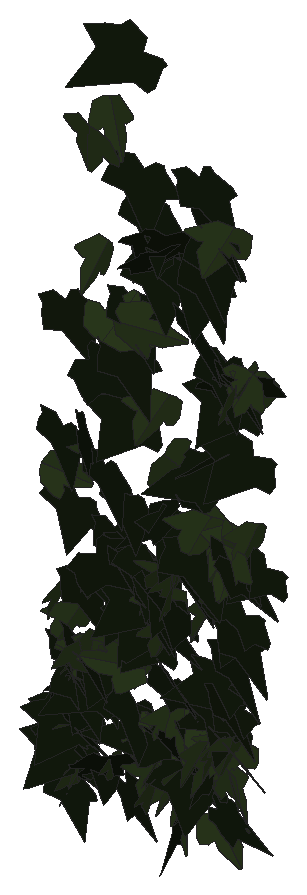
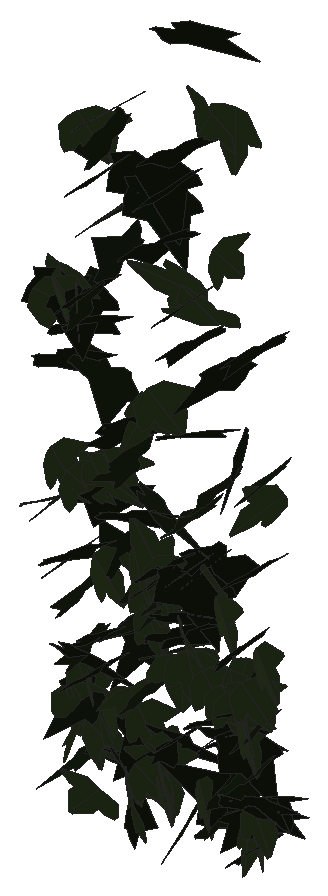
# SketchUp Ruby script. Lengths in inches.
U = 1.inch
M = Sketchup.active_model
def pt(a) = Geom::Point3d.new(a.map { |v| v * U })
def face(e, loops, mat)
  f = e.add_face(loops[0].map { |a| pt(a) })
  loops[1..].each { |l| e.add_face(l.map { |a| pt(a) }).erase! }
  f.material = f.back_material = mat if mat
  f
end
# faces: each face lists its corners as indices into pts; further lists are holes
def faces(e, pts, list, mat = nil) = list.each { |f| face(e, (f[0].is_a?(Array) ? f : [f]).map { |l| l.map { |i| pts[i] } }, mat) }
# xy, xz, yz: faces in a plane at the given z, y or x. An outline is a flat list of corners, or four numbers for a rectangle; further outlines are holes
def ring(l) = l.size == 4 ? [[l[0], l[1]], [l[2], l[1]], [l[2], l[3]], [l[0], l[3]]] : l.each_slice(2).to_a
def flat(e, list, mat, &to3) = list.each { |f| face(e, (f[0].is_a?(Array) ? f : [f]).map { |l| ring(l).map { |u, v| to3.(u, v) } }, mat) }
def xy(e, z, list, mat = nil) = flat(e, list, mat) { |x, y| [x, y, z] }
def xz(e, y, list, mat = nil) = flat(e, list, mat) { |x, z| [x, y, z] }
def yz(e, x, list, mat = nil) = flat(e, list, mat) { |y, z| [x, y, z] }
def lines(e, pts, list) = list.each { |a, b| e.add_line(pt(pts[a]), pt(pts[b])) }
# prism: a flat outline (further loops are holes) pulled along v
def prism(e, loops, v, mat = nil)
  f = face(e, loops, mat); d = Geom::Vector3d.new(v.map { |x| x * U })
  f.pushpull(f.normal.samedirection?(d) ? d.length : -d.length)
end
def box(e, o, s, mat = nil) = prism(e, [[o, [o[0] + s[0], o[1], o[2]], [o[0] + s[0], o[1] + s[1], o[2]], [o[0], o[1] + s[1], o[2]]]], [0, 0, s[2]], mat)
def at(x, y, z, deg = 0) = Geom::Transformation.translation(pt([x, y, z])) * Geom::Transformation.rotation(ORIGIN, Z_AXIS, deg.degrees)
def axes(o, x, y, z) = Geom::Transformation.new([*x, 0, *y, 0, *z, 0, *pt(o).to_a, 1])
def part(name) = M.definitions.add(name)
# library, detail: a bought-in or finely detailed component or shape, given as its bounding box
def library(name, o, s) = part(name).tap { |d| box(d.entities, o, s) }
def detail(e, o, s) = box(e.add_group.entities, o, s)
def put(e, d, t, mat = nil) = e.add_instance(d, t).tap { |i| i.material = mat if mat }
def group(e, t, mat = nil) = e.add_group.tap { |g| g.transformation = t; g.material = mat if mat }.entities
root = M.entities
M.materials.add("1026 AP 7946 SUNNY SIDE UP").color = [254, 231, 186]
M.materials.add("efeu1").color = [18, 25, 13]
M.materials.add("efeu2").color = [43, 57, 29]
c1 = part("ivyleaf_10")
p = [[0,0.5,-0.03],[-0.0625,2.02,-0.43],[-0.19,2.01,-0.46],[-0.54,1.05,-0.29],[-0.52,0.625,-0.18],[-0.83,0.76,-0.28],
  [-1.16,0.64,-0.33],[-1.15,0.33,-0.24],[-0.77,-0.39,0.02],[-0.3,-0.51,0.16],[0.04,-0.48,0.23],[-0.02,2.01,-0.4375],
  [-0.06,2.01,-0.43],[0.04,-0.49,0.23],[0.67,-0.49,0.14],[1.38,0.36,-0.2],[1.375,0.51,-0.24],[0.81,0.65,-0.19],
  [0.62,0.59,-0.15],[0.6,1.09,-0.28],[0.5,1.23,-0.31]]
faces(c1.entities,p,[[0,1,2,3,4,5,6,7,8,9,10],[11,12,0,13,14,15,16,17,18,19,20]],"efeu2")
c2 = part("ivyleaf_9")
p = [[1.54,2.16,1.25],[1.36,2.04,1.19],[-0.21,0.99,0.68],[-0.71,1.11,0.82],[-0.85,0.86,0.67],[-0.8,0.17,0.21],
  [-0.9,-0.01,0.1],[-0.67,-0.16,-0.02],[-0.08,-0.08,-0.05],[-0.03,-0.6,-0.4],[0.65,-0.88,-0.66],[0.83,-0.6,-0.49],
  [1.29,-0.42,-0.43],[1.8125,-0.07,-0.26],[1.21,0.44,0.15]]
faces(c2.entities,p,[[0,1,2,3,4,5,6,7,8,9,10,11,12,13,14]],"efeu1")
put(root,c1,axes([101.69,212.74,270.89],[0.06135,-0.27032,0.02668],[-0.00128,-0.02784,-0.28149],[0.42724,0.03874,-0.00467]),"1026 AP 7946 SUNNY SIDE UP")
put(root,c1,axes([101.78,212.89,270.46],[-0.14028,-0.22247,0.12848],[-0.01761,-0.1299,-0.24525],[0.40163,-0.0834,0.03412]),"1026 AP 7946 SUNNY SIDE UP")
put(root,c1,axes([101.77,212.74,268.71],[-0.10551,-0.24929,0.03591],[-0.00372,-0.03692,-0.26607],[0.3961,-0.06675,0.00707]),"1026 AP 7946 SUNNY SIDE UP")
put(root,c2,axes([101.83,212.91,268.95],[-0.3637,-0.12653,-0.00356],[0.02195,-0.01985,-0.27059],[0.19779,-0.23047,0.02349]),"1026 AP 7946 SUNNY SIDE UP")
put(root,c2,axes([101.8,212.74,268.9],[-0.27725,-0.1857,0.05475],[-0.00052,-0.07305,-0.25936],[0.30418,-0.16938,0.04946]),"1026 AP 7946 SUNNY SIDE UP")
put(root,c2,axes([101.98,212.71,269.62],[-0.03704,0.24109,-0.13395],[0.01426,-0.13112,-0.2503],[-0.43149,-0.02503,0.00323]),"1026 AP 7946 SUNNY SIDE UP")
put(root,c2,axes([101.98,212.58,268.64],[-0.37617,-0.13286,0.02716],[-0.01943,-0.0334,-0.28111],[0.21233,-0.23844,0.02238]),"1026 AP 7946 SUNNY SIDE UP")
put(root,c1,axes([101.9,212.79,269.84],[0.04693,-0.26813,-0.00958],[-0.00217,0.00768,-0.27789],[0.42178,0.02988,-0.00036]),"1026 AP 7946 SUNNY SIDE UP")
put(root,c1,axes([101.88,212.79,269.89],[0.1707,-0.24564,-0.02935],[0.02305,0.03594,-0.27498],[0.38791,0.10596,0.02926]),"1026 AP 7946 SUNNY SIDE UP")
put(root,c2,axes([101.73,212.71,268.71],[-0.02517,-0.20002,-0.19155],[0.04813,0.18262,-0.2053],[0.42549,-0.03249,0.01189]),"1026 AP 7946 SUNNY SIDE UP")
put(root,c2,axes([101.8,212.91,272.125],[-0.09531,-0.25363,0.10029],[-0.01045,-0.0998,-0.26874],[0.42786,-0.05893,0.01578]),"1026 AP 7946 SUNNY SIDE UP")
put(root,c2,axes([101.71,212.81,269.95],[0.13023,-0.25618,0.02363],[0.01274,-0.02302,-0.2775],[0.40445,0.08322,0.00113]),"1026 AP 7946 SUNNY SIDE UP")
put(root,c2,axes([101.75,212.67,273.29],[0.03354,-0.2698,0.08948],[0.00406,-0.08845,-0.2793],[0.4464,0.02108,-0.00418]),"1026 AP 7946 SUNNY SIDE UP")
put(root,c1,axes([101.86,212.35,272.87],[0.04364,0.15747,0.25361],[0.0374,0.24435,-0.16295],[-0.45679,0.03505,0.01088]),"1026 AP 7946 SUNNY SIDE UP")
put(root,c2,axes([101.8,212.6875,275.19],[0.07897,-0.27599,-0.09413],[-0.00818,0.09027,-0.28826],[0.45629,0.04939,0.01113]),"1026 AP 7946 SUNNY SIDE UP")
put(root,c2,axes([101.89,212.92,269.2],[-0.08827,-0.19579,0.17314],[0.01766,-0.1748,-0.20558],[0.40649,-0.03492,0.04653]),"1026 AP 7946 SUNNY SIDE UP")
put(root,c1,axes([102.03,212.56,268.31],[-0.0215,-0.23701,-0.10847],[0.04144,0.10228,-0.24321],[0.40483,-0.02306,0.01913]),"1026 AP 7946 SUNNY SIDE UP")
put(root,c2,axes([101.94,212.5625,268.1],[0.03053,-0.25633,-0.00335],[0.00157,0.00188,-0.26482],[0.40307,0.01941,0.00128]),"1026 AP 7946 SUNNY SIDE UP")
put(root,c1,axes([102.13,212.76,270.15],[-0.17048,-0.23168,0.08225],[0.01784,-0.09335,-0.25947],[0.38558,-0.09811,0.04837]),"1026 AP 7946 SUNNY SIDE UP")
put(root,c2,axes([101.93,212.81,271.04],[0.11093,-0.25844,-0.07029],[-0.03099,0.06383,-0.2756],[0.41857,0.07322,-0.00177]),"1026 AP 7946 SUNNY SIDE UP")
put(root,c1,axes([102.17,212.34,268.34],[0.12124,-0.25247,-0.11776],[-0.0597,0.10641,-0.27129],[0.43074,0.08581,-0.00445]),"1026 AP 7946 SUNNY SIDE UP")
put(root,c2,axes([101.98,212.54,269.04],[0.35668,-0.12337,-0.05003],[-0.04728,0.04444,-0.26457],[0.20263,0.22753,0.02632]),"1026 AP 7946 SUNNY SIDE UP")
put(root,c1,axes([102.27,212.7,270.17],[-0.23676,-0.18864,0.11946],[-0.03519,-0.12779,-0.24261],[0.34729,-0.14155,0.05686]),"1026 AP 7946 SUNNY SIDE UP")
put(root,c2,axes([102.4,212.65,269.64],[-0.36478,-0.09423,0.08935],[-0.10082,-0.07113,-0.25515],[0.17498,-0.23743,0.03925]),"1026 AP 7946 SUNNY SIDE UP")
put(root,c2,axes([102.09,212.65,269.68],[-0.02916,-0.26015,-0.04824],[0.04171,0.04339,-0.26738],[0.41313,-0.02274,0.02359]),"1026 AP 7946 SUNNY SIDE UP")
put(root,c2,axes([102.03,212.63,270.2],[0.15936,-0.23666,0.08942],[0.03797,-0.08546,-0.26549],[0.39528,0.10362,-0.01055]),"1026 AP 7946 SUNNY SIDE UP")
put(root,c2,axes([102.27,212.39,273.54],[0.22148,-0.10384,-0.24752],[-0.31208,0.13449,-0.1794],[0.26702,0.24331,-0.00436]),"1026 AP 7946 SUNNY SIDE UP")
put(root,c1,axes([102.28,212.34,270.35],[-0.11431,-0.25679,-0.12796],[0.06515,0.1158,-0.27416],[0.44278,-0.08333,0.0073]),"1026 AP 7946 SUNNY SIDE UP")
put(root,c1,axes([102.33,212.72,271.36],[0.069,-0.27178,-0.03272],[-0.02057,0.02848,-0.28331],[0.42949,0.04503,-0.00831]),"1026 AP 7946 SUNNY SIDE UP")
put(root,c1,axes([102.4,212.45,278.05],[-0.44421,0.11256,0.07978],[-0.12711,0.00388,-0.31216],[-0.17249,-0.29273,0.02458]),"1026 AP 7946 SUNNY SIDE UP")
put(root,c2,axes([102.17,212.89,269.79],[0.07347,-0.26324,0.00593],[-0.00478,-0.0079,-0.27543],[0.41405,0.04662,-0.00423]),"1026 AP 7946 SUNNY SIDE UP")
put(root,c2,axes([102.3125,212.92,269.93],[-0.19991,-0.2279,0.06311],[0.01017,-0.07436,-0.26598],[0.37146,-0.12062,0.04124]),"1026 AP 7946 SUNNY SIDE UP")
put(root,c1,axes([102.48,212.79,270.33],[-0.14945,-0.23602,0.10223],[-0.02521,-0.10158,-0.26179],[0.40263,-0.09397,0.02156]),"1026 AP 7946 SUNNY SIDE UP")
put(root,c1,axes([102.42,212.63,276.22],[-0.04992,-0.20654,0.21954],[0.10362,-0.21503,-0.20471],[0.45635,0.02623,0.0705]),"1026 AP 7946 SUNNY SIDE UP")
put(root,c2,axes([102.32,212.79,268.39],[-0.04008,-0.20176,0.16635],[0.05283,-0.1646,-0.20592],[0.40404,0.00151,0.04343]),"1026 AP 7946 SUNNY SIDE UP")
put(root,c2,axes([102.39,212.47,274.6],[0.1456,-0.12586,-0.25877],[-0.09406,0.24883,-0.15014],[0.43061,0.09691,0.0547]),"1026 AP 7946 SUNNY SIDE UP")
put(root,c1,axes([102.64,212.7,268.6875],[0.05602,-0.26314,-0.02053],[0.00844,0.01932,-0.27332],[0.41469,0.03515,0.00834]),"1026 AP 7946 SUNNY SIDE UP")
put(root,c1,axes([102.39,212.85,278.25],[0.3549,-0.08919,0.19583],[0.27093,-0.08212,-0.25027],[0.18994,0.28377,-0.00891]),"1026 AP 7946 SUNNY SIDE UP")
put(root,c2,axes([102.44,212.7,272.94],[0.06881,-0.27024,0.07645],[0.01432,-0.07525,-0.28245],[0.44106,0.0446,-0.00276]),"1026 AP 7946 SUNNY SIDE UP")
put(root,c2,axes([102.39,212.39,268.52],[0.20207,0.22585,-0.10278],[0.06109,0.09403,0.26797],[0.38422,-0.13373,0.01145]),"1026 AP 7946 SUNNY SIDE UP")
put(root,c2,axes([102.49,212.85,271.93],[0.08598,-0.27536,0.00093],[-0.00806,-0.00353,-0.28918],[0.43293,0.05462,-0.00557]),"1026 AP 7946 SUNNY SIDE UP")
put(root,c2,axes([102.91,212.82,279.29],[-0.43546,-0.10836,0.10054],[-0.12951,-0.05821,-0.30579],[0.19,-0.28801,0.02198]),"1026 AP 7946 SUNNY SIDE UP")
put(root,c2,axes([102.82,212.69,271.6],[0.07705,0.24379,-0.12181],[-0.07714,-0.11161,-0.25568],[-0.41997,0.06523,0.02461]),"1026 AP 7946 SUNNY SIDE UP")
put(root,c1,axes([102.76,212.8125,270.49],[-0.24342,-0.21776,0.03459],[-0.00974,-0.03823,-0.27492],[0.34663,-0.154,0.01657]),"1026 AP 7946 SUNNY SIDE UP")
put(root,c1,axes([103,212.5,270.22],[0.05178,-0.01705,-0.28476],[-0.4333,-0.02877,-0.03217],[-0.04184,0.27679,-0.01924]),"1026 AP 7946 SUNNY SIDE UP")
put(root,c2,axes([102.7,212.95,270.98],[-0.19313,-0.22883,0.0831],[-0.04562,-0.07738,-0.26778],[0.37947,-0.12577,0.0101]),"1026 AP 7946 SUNNY SIDE UP")
put(root,c2,axes([102.78,212.9,273.73],[-0.29732,-0.19703,0.08795],[0.00211,-0.11621,-0.2704],[0.33834,-0.17242,0.07896]),"1026 AP 7946 SUNNY SIDE UP")
put(root,c2,axes([102.6,212.36,271.81],[0.04069,-0.08823,-0.30605],[-0.01684,0.29719,-0.09031],[0.48626,0.01768,0.02248]),"1026 AP 7946 SUNNY SIDE UP")
put(root,c1,axes([102.71,212.46,275.18],[0.43753,0.03042,-0.10492],[0.1359,0.10211,0.27483],[0.09771,-0.27822,0.08753]),"1026 AP 7946 SUNNY SIDE UP")
put(root,c2,axes([102.74,212.83,272.52],[-0.00952,-0.26013,0.11227],[0.03698,-0.11057,-0.26756],[0.44284,0.00364,0.02476]),"1026 AP 7946 SUNNY SIDE UP")
put(root,c1,axes([102.95,212.76,270.37],[-0.35485,-0.14876,0.01091],[0.00408,-0.02465,-0.27767],[0.23456,-0.22462,0.02134]),"1026 AP 7946 SUNNY SIDE UP")
put(root,c1,axes([102.77,212.89,270.92],[0.25505,-0.14869,0.16337],[0.16943,-0.11806,-0.22706],[0.29799,0.19439,-0.01072]),"1026 AP 7946 SUNNY SIDE UP")
put(root,c2,axes([103.03,212.82,271.07],[-0.36514,-0.1255,0.06824],[-0.0435,-0.08588,-0.2652],[0.21939,-0.2259,0.06099]),"1026 AP 7946 SUNNY SIDE UP")
put(root,c2,axes([102.85,212.66,268.28],[0.21151,-0.18498,-0.13962],[-0.15943,0.0916,-0.23376],[0.32232,0.16669,-0.02401]),"1026 AP 7946 SUNNY SIDE UP")
put(root,c2,axes([102.76,212.79,271.82],[0.10918,-0.27006,-0.01974],[0.01333,0.02036,-0.28682],[0.42534,0.06868,0.01406]),"1026 AP 7946 SUNNY SIDE UP")
put(root,c2,axes([102.88,212.78,269.46],[-0.02822,-0.26249,0.05753],[0.00438,-0.05764,-0.2713],[0.42245,-0.01694,0.00666]),"1026 AP 7946 SUNNY SIDE UP")
put(root,c2,axes([102.83,212.81,275.49],[0.05451,-0.29331,0.00687],[0.00378,-0.00811,-0.30431],[0.46137,0.03472,0.00168]),"1026 AP 7946 SUNNY SIDE UP")
put(root,c1,axes([103.03,212.65,271.64],[-0.40153,-0.10579,-0.02683],[0.05106,-0.01215,-0.28378],[0.16329,-0.25633,0.02276]),"1026 AP 7946 SUNNY SIDE UP")
put(root,c2,axes([103.36,212.63,269.18],[-0.33141,0.05637,0.1632],[-0.25567,-0.00559,-0.22129],[-0.06549,-0.26341,0.03801]),"1026 AP 7946 SUNNY SIDE UP")
put(root,c2,axes([102.875,212.6,274.875],[0.03031,-0.28884,-0.05501],[0.00831,0.0522,-0.29779],[0.46134,0.01804,0.00898]),"1026 AP 7946 SUNNY SIDE UP")
put(root,c2,axes([103.0625,212.82,270.83],[-0.24301,-0.21252,0.05917],[-0.02465,-0.06084,-0.27007],[0.34578,-0.1537,0.02233]),"1026 AP 7946 SUNNY SIDE UP")
put(root,c2,axes([103.12,212.88,270.54],[-0.24492,-0.18058,0.12835],[-0.00566,-0.1518,-0.23031],[0.34584,-0.13037,0.08712]),"1026 AP 7946 SUNNY SIDE UP")
put(root,c1,axes([103.21,212.91,274.07],[-0.18327,-0.23173,0.16577],[-0.00533,-0.1743,-0.26002],[0.44475,-0.09757,0.06519]),"1026 AP 7946 SUNNY SIDE UP")
put(root,c2,axes([103.03,212.77,277.57],[-0.08645,-0.30026,-0.0048],[0.01446,0.00132,-0.31433],[0.47193,-0.05504,0.00875]),"1026 AP 7946 SUNNY SIDE UP")
put(root,c2,axes([103.14,212.8,271.72],[-0.10227,-0.26863,0.03369],[-0.01027,-0.03364,-0.28493],[0.42569,-0.06535,0.00122]),"1026 AP 7946 SUNNY SIDE UP")
put(root,c2,axes([103.125,212.84,277],[-0.01325,-0.29822,0.04803],[-0.01442,-0.04806,-0.30753],[0.47482,-0.00978,-0.008]),"1026 AP 7946 SUNNY SIDE UP")
put(root,c2,axes([103.46,212.73,272.51],[-0.34468,0.15573,-0.07789],[0.05017,-0.08496,-0.2729],[-0.26816,-0.21606,0.04906]),"1026 AP 7946 SUNNY SIDE UP")
put(root,c1,axes([103.29,212.68,268.78],[0.11243,-0.24999,-0.04319],[-0.00555,0.0411,-0.26751],[0.39818,0.07116,0.00847]),"1026 AP 7946 SUNNY SIDE UP")
put(root,c1,axes([103.35,212.65,268.93],[0.29361,0.19363,0.02521],[-0.04834,-0.00273,0.27632],[0.30283,-0.18816,0.01967]),"1026 AP 7946 SUNNY SIDE UP")
put(root,c1,axes([103.47,212.63,268.68],[-0.33867,-0.13012,0.10406],[-0.10974,-0.07985,-0.25787],[0.2354,-0.22443,0.0295]),"1026 AP 7946 SUNNY SIDE UP")
put(root,c1,axes([103.4,212.91,268.79],[-0.07399,-0.20754,0.15201],[-0.02877,-0.14811,-0.21974],[0.40045,-0.04899,0.0123]),"1026 AP 7946 SUNNY SIDE UP")
put(root,c1,axes([103.37,212.54,268.56],[0.04674,-0.26378,-0.04392],[0.00198,0.04153,-0.27315],[0.41977,0.02917,0.00618]),"1026 AP 7946 SUNNY SIDE UP")
put(root,c2,axes([103.27,212.84,276.2],[-0.08256,-0.29492,-0.01198],[0.00923,0.00907,-0.30851],[0.4639,-0.05267,0.00401]),"1026 AP 7946 SUNNY SIDE UP")
put(root,c1,axes([103.43,212.75,271.31],[-0.19273,-0.23128,0.0848],[0.01668,-0.09832,-0.26469],[0.38634,-0.11113,0.05373]),"1026 AP 7946 SUNNY SIDE UP")
put(root,c1,axes([103.44,212.75,270.89],[-0.07736,-0.2662,0.05554],[0.00299,-0.05666,-0.27894],[0.42754,-0.04777,0.012]),"1026 AP 7946 SUNNY SIDE UP")
put(root,c2,axes([103.53,212.43,276.65],[0.02106,0.28843,-0.09389],[-0.02432,-0.09209,-0.29779],[-0.47579,0.01747,0.01106]),"1026 AP 7946 SUNNY SIDE UP")
put(root,c2,axes([103.22,212.73,271.28],[0.10285,-0.25802,0.08345],[0.02789,-0.08058,-0.27468],[0.42502,0.06773,-0.00217]),"1026 AP 7946 SUNNY SIDE UP")
put(root,c1,axes([103.07,212.44,275.43],[0.03117,-0.0313,-0.30798],[0.45926,-0.06803,0.02691],[-0.11049,-0.2916,0.02496]),"1026 AP 7946 SUNNY SIDE UP")
put(root,c1,axes([103.49,212.8125,269.52],[-0.12149,-0.24235,0.08202],[0.01134,-0.08664,-0.26053],[0.40163,-0.07086,0.03216]),"1026 AP 7946 SUNNY SIDE UP")
put(root,c2,axes([103.39,212.83,271.375],[-0.08117,-0.23385,0.13878],[-0.0439,-0.13315,-0.24749],[0.42313,-0.05868,0.00094]),"1026 AP 7946 SUNNY SIDE UP")
put(root,c1,axes([103.44,212.68,271.61],[-0.08248,-0.27853,0.0477],[0.02637,0.04555,0.29214],[-0.4436,0.05449,0.0085]),"1026 AP 7946 SUNNY SIDE UP")
put(root,c1,axes([103.56,212.75,271.7],[-0.02323,-0.27853,-0.01455],[0.01179,0.01216,-0.28719],[0.43825,-0.01509,0.00696]),"1026 AP 7946 SUNNY SIDE UP")
put(root,c2,axes([103.36,212.93,269.9],[0.04086,-0.24836,0.09861],[0.02995,-0.09561,-0.25767],[0.41825,0.03111,0.00882]),"1026 AP 7946 SUNNY SIDE UP")
put(root,c2,axes([103.67,212.42,276.95],[0.1381,0.23816,-0.17214],[-0.10746,-0.15423,-0.26224],[-0.44592,0.11092,0.00988]),"1026 AP 7946 SUNNY SIDE UP")
put(root,c2,axes([103.43,212.625,269.24],[0.41514,0.01168,-0.05671],[-0.08511,-0.02064,-0.27175],[-0.02457,0.26891,-0.01681]),"1026 AP 7946 SUNNY SIDE UP")
put(root,c1,axes([103.65,212.76,268.625],[0.05411,-0.20371,0.1725],[0.02748,-0.1679,-0.21364],[0.41488,0.03769,-0.00835]),"1026 AP 7946 SUNNY SIDE UP")
put(root,c2,axes([103.43,212.66,270.96],[0.28502,-0.18528,-0.08996],[-0.04248,0.09258,-0.26277],[0.31855,0.17813,0.04545]),"1026 AP 7946 SUNNY SIDE UP")
put(root,c2,axes([103.65,212.91,272.32],[-0.29916,-0.2042,0.01976],[0.04928,-0.05632,-0.28086],[0.31888,-0.18286,0.06194]),"1026 AP 7946 SUNNY SIDE UP")
put(root,c1,axes([103.68,212.49,271.59],[0.12659,-0.24749,-0.09281],[0.01776,0.09592,-0.26464],[0.413,0.07173,0.03983]),"1026 AP 7946 SUNNY SIDE UP")
put(root,c1,axes([103.67,212.48,273.61],[-0.09654,-0.21719,-0.20357],[0.1367,0.17807,-0.22986],[0.43964,-0.10306,0.02677]),"1026 AP 7946 SUNNY SIDE UP")
put(root,c2,axes([103.59,212.73,271.21],[-0.05656,-0.20957,0.18192],[0.03802,-0.18102,-0.21585],[0.43045,-0.01155,0.04297]),"1026 AP 7946 SUNNY SIDE UP")
put(root,c1,axes([103.64,212.79,268.13],[0.23491,-0.16071,0.14874],[0.20458,-0.07458,-0.22323],[0.2724,0.1946,0.03937]),"1026 AP 7946 SUNNY SIDE UP")
put(root,c2,axes([103.76,212.67,268.09],[-0.10388,0.04542,-0.26171],[0.27917,-0.18268,-0.0822],[-0.29505,-0.18884,0.01437]),"1026 AP 7946 SUNNY SIDE UP")
put(root,c2,axes([103.61,212.81,273.05],[0.27513,-0.22199,-0.01518],[-0.00518,0.01455,-0.29103],[0.34966,0.17489,0.00763]),"1026 AP 7946 SUNNY SIDE UP")
put(root,c2,axes([104.04,212.84,273.25],[-0.22673,-0.11551,0.2208],[-0.23821,-0.15341,-0.19049],[0.30087,-0.20851,0.01558]),"1026 AP 7946 SUNNY SIDE UP")
put(root,c1,axes([103.84,212.63,269.64],[0.13847,0.2518,-0.06233],[-0.01963,-0.06122,-0.27503],[-0.40726,0.08856,-0.00794]),"1026 AP 7946 SUNNY SIDE UP")
put(root,c2,axes([103.8,212.36,270.38],[0.36882,-0.10114,-0.14433],[-0.20859,0.04444,-0.26267],[0.17296,0.26927,-0.00902]),"1026 AP 7946 SUNNY SIDE UP")
put(root,c2,axes([103.91,212.68,268.79],[-0.248,-0.20655,-0.06048],[0.13892,0.00247,-0.25864],[0.3072,-0.16787,0.06814]),"1026 AP 7946 SUNNY SIDE UP")
put(root,c2,axes([104.05,212.75,268.88],[-0.30218,0.04433,-0.17804],[0.23837,-0.09407,-0.19878],[-0.14868,-0.24091,0.04318]),"1026 AP 7946 SUNNY SIDE UP")
put(root,c1,axes([104.08,212.875,271.42],[0.03623,-0.27131,0.11827],[0.0213,-0.1156,-0.28116],[0.46369,0.02651,0.00368]),"1026 AP 7946 SUNNY SIDE UP")
put(root,c1,axes([104.39,212.71,272.58],[-0.06775,0.04283,0.28783],[-0.444,-0.01156,-0.04314],[0.0079,-0.28222,0.04376]),"1026 AP 7946 SUNNY SIDE UP")
put(root,c1,axes([104.2,212.61,272.73],[-0.28858,-0.18173,0.11236],[-0.04467,-0.12319,-0.25898],[0.3311,-0.17501,0.06299]),"1026 AP 7946 SUNNY SIDE UP")
put(root,c2,axes([103.9,212.76,271.51],[0.02036,-0.15971,0.22617],[0.11692,-0.21023,-0.16263],[0.41177,0.06759,0.035]),"1026 AP 7946 SUNNY SIDE UP")
put(root,c1,axes([104.14,212.57,269.33],[0.02841,-0.23381,0.12838],[0.02586,-0.12501,-0.24224],[0.41679,0.02369,0.00628]),"1026 AP 7946 SUNNY SIDE UP")
put(root,c2,axes([104.04,212.64,276.28],[-0.07181,-0.27273,0.115],[0.012,-0.11557,-0.28442],[0.46415,-0.03921,0.02515]),"1026 AP 7946 SUNNY SIDE UP")
put(root,c1,axes([104.21,212.83,269.1],[-0.00692,-0.243,0.15578],[-0.0023,-0.15259,-0.25126],[0.45117,-0.00451,0.00111]),"1026 AP 7946 SUNNY SIDE UP")
put(root,c2,axes([104,212.84,276.37],[0.06041,-0.29811,0.01217],[-0.00078,-0.01368,-0.30972],[0.46923,0.03836,-0.00208]),"1026 AP 7946 SUNNY SIDE UP")
put(root,c2,axes([104.01,212.75,277.78],[0.11943,-0.28966,-0.06466],[0.02903,0.06762,-0.30607],[0.46459,0.07024,0.03575]),"1026 AP 7946 SUNNY SIDE UP")
put(root,c2,axes([104.39,212.78,270.25],[-0.2765,-0.07591,0.20093],[-0.18603,-0.17471,-0.18056],[0.27223,-0.19649,0.0807]),"1026 AP 7946 SUNNY SIDE UP")
put(root,c2,axes([104.11,212.57,272.3125],[-0.11074,-0.2558,-0.13358],[0.07411,0.11986,-0.27233],[0.44376,-0.08385,0.01214]),"1026 AP 7946 SUNNY SIDE UP")
put(root,c2,axes([104.01,212.59,275.61],[0.11832,-0.23657,0.16993],[0.08755,-0.15677,-0.25661],[0.44618,0.0935,0.00529]),"1026 AP 7946 SUNNY SIDE UP")
put(root,c1,axes([104.38,212.69,269.04],[-0.34949,0.13487,0.06655],[-0.1369,-0.02421,-0.25975],[-0.19055,-0.22998,0.06455]),"1026 AP 7946 SUNNY SIDE UP")
put(root,c2,axes([104.05,212.76,277.34],[0.22104,-0.26319,0.05752],[0.01593,-0.05946,-0.30713],[0.42325,0.13969,-0.01848]),"1026 AP 7946 SUNNY SIDE UP")
put(root,c2,axes([104.4,212.32,273.8125],[0.09798,0.25942,0.11516],[-0.03302,0.11693,-0.27039],[-0.44203,0.04877,0.04573]),"1026 AP 7946 SUNNY SIDE UP")
put(root,c2,axes([104.64,212.79,270.01],[-0.41274,0.03403,0.06547],[-0.10535,-0.02855,-0.27032],[-0.0411,-0.26852,0.03542]),"1026 AP 7946 SUNNY SIDE UP")
put(root,c2,axes([104.24,212.75,276.78],[0.00631,-0.29902,0.04294],[0.00244,-0.04336,-0.30833],[0.47509,0.0042,0.00101]),"1026 AP 7946 SUNNY SIDE UP")
put(root,c2,axes([104.3,212.89,269.84],[-0.0884,-0.26662,0.10095],[-0.01682,-0.09937,-0.28113],[0.44717,-0.05645,0.00939]),"1026 AP 7946 SUNNY SIDE UP")
put(root,c1,axes([104.54,212.78,269.42],[-0.31636,-0.13775,0.1179],[-0.08392,-0.11935,-0.24369],[0.26963,-0.19877,0.06248]),"1026 AP 7946 SUNNY SIDE UP")
put(root,c1,axes([104.44,212.57,269.52],[0.0844,-0.25787,0.04554],[0.00455,-0.04603,-0.27154],[0.41177,0.05336,-0.00634]),"1026 AP 7946 SUNNY SIDE UP")
put(root,c1,axes([104.49,212.86,272.49],[-0.12632,-0.20436,0.21107],[0.04196,-0.21809,-0.2134],[0.45438,-0.03667,0.07838]),"1026 AP 7946 SUNNY SIDE UP")
put(root,c2,axes([104.52,212.83,274.64],[-0.28521,-0.2151,0.08558],[-0.03989,-0.08797,-0.28803],[0.36107,-0.17963,0.03577]),"1026 AP 7946 SUNNY SIDE UP")
put(root,c1,axes([104.26,212.78,268.15],[0.33288,0.00191,0.1594],[0.243,0.01035,-0.21792],[-0.01202,0.26201,0.00899]),"1026 AP 7946 SUNNY SIDE UP")
put(root,c2,axes([104.38,212.8,275.11],[0.01001,-0.29475,0.0142],[-0.00943,-0.01559,-0.30375],[0.46401,0.00604,-0.00648]),"1026 AP 7946 SUNNY SIDE UP")
put(root,c2,axes([104.3,212.85,275.06],[0.253,-0.24112,0.05159],[0.01395,-0.05574,-0.298],[0.38743,0.15947,-0.02297]),"1026 AP 7946 SUNNY SIDE UP")
put(root,c1,axes([104.64,212.52,277.26],[-0.26294,-0.20856,0.15026],[-0.03111,-0.16468,-0.26477],[0.40005,-0.14988,0.07817]),"1026 AP 7946 SUNNY SIDE UP")
put(root,c2,axes([104.41,212.7,269.47],[0.37524,-0.08659,-0.09415],[-0.12677,0.04395,-0.26093],[0.15131,0.25156,0.01487]),"1026 AP 7946 SUNNY SIDE UP")
put(root,c2,axes([104.39,212.73,270.14],[0.18281,-0.24477,0.00129],[-0.01295,-0.00684,-0.279],[0.38469,0.11609,-0.01001]),"1026 AP 7946 SUNNY SIDE UP")
put(root,c1,axes([104.64,212.56,269.61],[-0.08709,-0.26187,0.01448],[0.0021,-0.01617,-0.2758],[0.41249,-0.05521,0.00446]),"1026 AP 7946 SUNNY SIDE UP")
put(root,c2,axes([104.42,212.85,272.48],[0.12259,-0.26688,-0.03797],[-0.00513,0.03585,-0.28613],[0.42328,0.07773,0.00753]),"1026 AP 7946 SUNNY SIDE UP")
put(root,c2,axes([104.71,212.66,275.03],[0.20862,0.22639,-0.13029],[-0.09371,-0.11312,-0.27093],[-0.39785,0.14535,-0.0045]),"1026 AP 7946 SUNNY SIDE UP")
put(root,c1,axes([104.64,212.68,268.95],[-0.13215,0.25346,0.01959],[-0.0187,0.01457,-0.27492],[-0.39906,-0.08461,0.00639]),"1026 AP 7946 SUNNY SIDE UP")
put(root,c1,axes([104.67,212.57,274.86],[0.10407,-0.2767,-0.08264],[0.03827,0.0858,-0.28938],[0.4507,0.05661,0.04365]),"1026 AP 7946 SUNNY SIDE UP")
put(root,c2,axes([104.64,212.85,271.39],[-0.18832,-0.23311,0.08491],[-0.01129,-0.08972,-0.26837],[0.38932,-0.11536,0.03329]),"1026 AP 7946 SUNNY SIDE UP")
put(root,c2,axes([104.51,212.53,268.55],[0.28159,-0.13514,-0.14321],[-0.08539,0.1457,-0.21834],[0.29175,0.17308,0.07432]),"1026 AP 7946 SUNNY SIDE UP")
put(root,c1,axes([104.62,212.57,272.36],[0.40908,-0.09915,0.03514],[0.03516,-0.03822,-0.28564],[0.16138,0.25966,-0.02685]),"1026 AP 7946 SUNNY SIDE UP")
put(root,c2,axes([104.52,212.69,270.84],[0.15749,-0.26211,0.01139],[-0.0042,-0.01444,-0.28904],[0.41259,0.0999,-0.00729]),"1026 AP 7946 SUNNY SIDE UP")
put(root,c1,axes([104.76,212.84,275.05],[0.14846,-0.27551,0.04078],[0.00394,-0.04261,-0.30005],[0.43799,0.09377,-0.01112]),"1026 AP 7946 SUNNY SIDE UP")
put(root,c1,axes([104.78,212.86,272.7],[-0.0565,-0.24891,0.12843],[0.04395,-0.12969,-0.25633],[0.43653,-0.01916,0.04243]),"1026 AP 7946 SUNNY SIDE UP")
put(root,c1,axes([104.92,212.9,274.92],[-0.11837,-0.14515,0.24593],[-0.10245,-0.23217,-0.16738],[0.42834,-0.09565,0.02793]),"1026 AP 7946 SUNNY SIDE UP")
put(root,c2,axes([104.92,212.65,273.97],[-0.33233,-0.18127,0.06396],[-0.05591,-0.05528,-0.28655],[0.29659,-0.21354,0.01766]),"1026 AP 7946 SUNNY SIDE UP")
put(root,c2,axes([104.65,212.61,272.3],[0.22045,-0.20149,-0.14105],[-0.07501,0.13088,-0.25007],[0.37461,0.14478,0.03293]),"1026 AP 7946 SUNNY SIDE UP")
put(root,c2,axes([104.87,213,272.13],[-0.26279,-0.17774,0.13026],[-0.01054,-0.15616,-0.23433],[0.34375,-0.14067,0.0924]),"1026 AP 7946 SUNNY SIDE UP")
put(root,c1,axes([104.88,212.58,275.12],[0.40861,-0.12898,-0.03025],[-0.0544,-0.00547,-0.29818],[0.20049,0.26138,-0.01927]),"1026 AP 7946 SUNNY SIDE UP")
put(root,c2,axes([104.71,212.64,271.26],[0.11599,-0.26275,-0.03778],[-0.00576,0.0355,-0.28087],[0.41679,0.07361,0.00663]),"1026 AP 7946 SUNNY SIDE UP")
